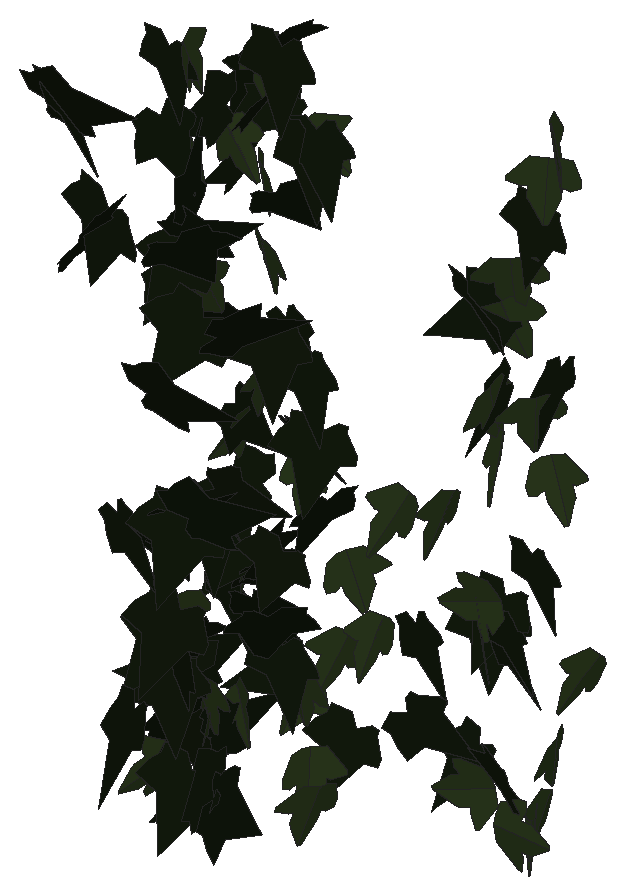
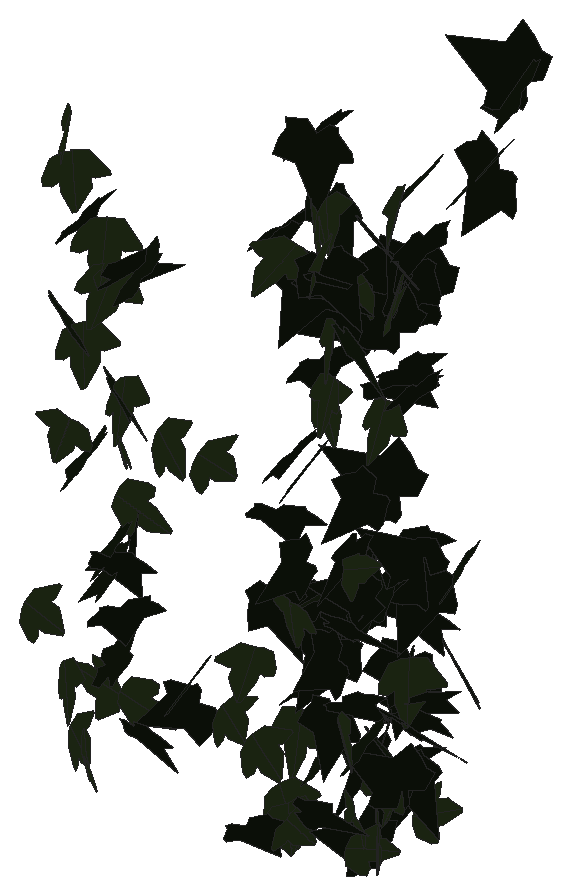
# SketchUp Ruby script. Lengths in inches.
U = 1.inch
M = Sketchup.active_model
def pt(a) = Geom::Point3d.new(a.map { |v| v * U })
def face(e, loops, mat)
  f = e.add_face(loops[0].map { |a| pt(a) })
  loops[1..].each { |l| e.add_face(l.map { |a| pt(a) }).erase! }
  f.material = f.back_material = mat if mat
  f
end
# faces: each face lists its corners as indices into pts; further lists are holes
def faces(e, pts, list, mat = nil) = list.each { |f| face(e, (f[0].is_a?(Array) ? f : [f]).map { |l| l.map { |i| pts[i] } }, mat) }
# xy, xz, yz: faces in a plane at the given z, y or x. An outline is a flat list of corners, or four numbers for a rectangle; further outlines are holes
def ring(l) = l.size == 4 ? [[l[0], l[1]], [l[2], l[1]], [l[2], l[3]], [l[0], l[3]]] : l.each_slice(2).to_a
def flat(e, list, mat, &to3) = list.each { |f| face(e, (f[0].is_a?(Array) ? f : [f]).map { |l| ring(l).map { |u, v| to3.(u, v) } }, mat) }
def xy(e, z, list, mat = nil) = flat(e, list, mat) { |x, y| [x, y, z] }
def xz(e, y, list, mat = nil) = flat(e, list, mat) { |x, z| [x, y, z] }
def yz(e, x, list, mat = nil) = flat(e, list, mat) { |y, z| [x, y, z] }
def lines(e, pts, list) = list.each { |a, b| e.add_line(pt(pts[a]), pt(pts[b])) }
# prism: a flat outline (further loops are holes) pulled along v
def prism(e, loops, v, mat = nil)
  f = face(e, loops, mat); d = Geom::Vector3d.new(v.map { |x| x * U })
  f.pushpull(f.normal.samedirection?(d) ? d.length : -d.length)
end
def box(e, o, s, mat = nil) = prism(e, [[o, [o[0] + s[0], o[1], o[2]], [o[0] + s[0], o[1] + s[1], o[2]], [o[0], o[1] + s[1], o[2]]]], [0, 0, s[2]], mat)
def at(x, y, z, deg = 0) = Geom::Transformation.translation(pt([x, y, z])) * Geom::Transformation.rotation(ORIGIN, Z_AXIS, deg.degrees)
def axes(o, x, y, z) = Geom::Transformation.new([*x, 0, *y, 0, *z, 0, *pt(o).to_a, 1])
def part(name) = M.definitions.add(name)
# library, detail: a bought-in or finely detailed component or shape, given as its bounding box
def library(name, o, s) = part(name).tap { |d| box(d.entities, o, s) }
def detail(e, o, s) = box(e.add_group.entities, o, s)
def put(e, d, t, mat = nil) = e.add_instance(d, t).tap { |i| i.material = mat if mat }
def group(e, t, mat = nil) = e.add_group.tap { |g| g.transformation = t; g.material = mat if mat }.entities
root = M.entities
M.materials.add("efeu1").color = [18, 25, 13]
M.materials.add("efeu2").color = [43, 57, 29]
c1 = part("ivyleaf_9")
p = [[1.54,2.16,1.25],[1.36,2.04,1.19],[-0.21,0.99,0.68],[-0.71,1.11,0.82],[-0.85,0.86,0.67],[-0.8,0.17,0.21],
  [-0.9,-0.01,0.1],[-0.67,-0.16,-0.02],[-0.08,-0.08,-0.05],[-0.03,-0.6,-0.4],[0.65,-0.88,-0.66],[0.83,-0.6,-0.49],
  [1.29,-0.42,-0.43],[1.8125,-0.07,-0.26],[1.21,0.44,0.15]]
faces(c1.entities,p,[[0,1,2,3,4,5,6,7,8,9,10,11,12,13,14]],"efeu1")
c2 = part("ivyleaf_10")
p = [[0,0.5,-0.03],[-0.0625,2.02,-0.43],[-0.19,2.01,-0.46],[-0.54,1.05,-0.29],[-0.52,0.625,-0.18],[-0.83,0.76,-0.28],
  [-1.16,0.64,-0.33],[-1.15,0.33,-0.24],[-0.77,-0.39,0.02],[-0.3,-0.51,0.16],[0.04,-0.48,0.23],[-0.02,2.01,-0.4375],
  [-0.06,2.01,-0.43],[0.04,-0.49,0.23],[0.67,-0.49,0.14],[1.38,0.36,-0.2],[1.375,0.51,-0.24],[0.81,0.65,-0.19],
  [0.62,0.59,-0.15],[0.6,1.09,-0.28],[0.5,1.23,-0.31]]
faces(c2.entities,p,[[0,1,2,3,4,5,6,7,8,9,10],[11,12,0,13,14,15,16,17,18,19,20]],"efeu2")
put(root,c1,axes([505.17,116.25,275.17],[0.52093,-0.38038,1.18336],[1.14923,-0.43079,-0.6189],[0.59847,1.15835,0.15843]))
put(root,c1,axes([506.65,117.58,270.4],[-0.10855,-1.09886,0.74671],[0.12021,-0.72463,-1.13718],[1.41254,-0.02278,0.15416]))
put(root,c1,axes([504.65,117.03,275.1],[0.77226,-0.95206,0.32614],[0.18154,-0.26586,-1.23805],[1.06724,0.73414,-0.0254]))
put(root,c1,axes([506.9375,115.67,270.03],[0.23492,1.04021,0.76758],[0.17346,0.72041,-1.10519],[-1.36652,0.27027,-0.00833]))
put(root,c1,axes([509.34,116.88,263.82],[0.67363,-0.32063,1.11659],[1.08327,-0.38796,-0.72651],[0.53942,1.17952,0.06457]))
put(root,c1,axes([506.99,118.65,248.56],[-1.05734,0.11517,-0.80677],[0.81643,-0.19168,-1.0218],[-0.22544,-1.23431,0.0834]))
put(root,c1,axes([508.26,120.65,256.49],[0.3412,-0.2438,1.2276],[1.23845,-0.31503,-0.38686],[0.40092,1.18062,0.15027]))
put(root,c1,axes([507.13,121.23,251.75],[-1.09872,-0.50946,-0.32223],[0.33647,0.06829,-1.18065],[0.54908,-1.06127,0.07871]))
put(root,c1,axes([507.28,121.79,244.67],[-0.50911,-1.02221,0.18292],[-0.05197,-0.17144,-1.17034],[1.119,-0.47303,0.02887]))
put(root,c1,axes([508.73,121.21,244.91],[-1.0834,0.6632,0.14675],[-0.1257,0.07982,-1.25066],[-0.72142,-1.00988,-0.00247]))
put(root,c1,axes([504.18,121.41,254.75],[0.73239,-0.84204,-0.25402],[-0.16045,0.19396,-1.12438],[0.93319,0.6942,0.00603]))
put(root,c1,axes([506.95,122.05,255.43],[-0.77344,-0.96925,-0.12279],[0.08584,0.08807,-1.25327],[1.05102,-0.72046,0.01199]))
put(root,c1,axes([509.58,120.73,264.65],[0.76725,0.40794,0.97112],[0.74256,0.64824,-0.83854],[-0.81224,0.97797,0.15074]))
put(root,c1,axes([507.34,121.01,267.73],[0.76991,1.02592,-0.02188],[-0.01175,-0.01805,-1.29926],[-1.10817,0.71296,-0.00142]))
put(root,c1,axes([509.17,120.96,244.51],[0.34449,-0.2086,-1.23135],[-0.81236,0.92096,-0.37949],[1.01288,0.80958,0.11443]))
put(root,c1,axes([505.78,122.6875,248.05],[-0.62327,-0.66376,-0.64536],[0.74275,0.16138,-0.8447],[0.64137,-0.83191,0.35107]))
put(root,c1,axes([506.74,123.05,263.35],[-0.90501,-0.82243,0.19368],[-0.0826,-0.18733,-1.21832],[0.90696,-0.83773,0.0823]))
put(root,c1,axes([506.62,121.84,249.64],[0.67569,-0.2485,-0.99126],[-0.8866,0.49246,-0.69393],[0.58789,1.02829,0.09278]))
put(root,c2,axes([504.74,123.16,243.67],[0.00953,-0.18123,1.04984],[0.07515,-1.00707,-0.18866],[1.1051,0.07005,0.00378]))
put(root,c1,axes([505.47,122.07,254.36],[0.56594,0.96324,-0.36059],[0.19221,0.29785,1.14033],[1.08881,-0.55326,-0.01388]))
put(root,c1,axes([505.34,122.18,254.23],[0.98085,0.6315,-0.27896],[-0.24823,-0.13925,-1.15029],[-0.69818,0.93668,0.01707]))
put(root,c1,axes([506.26,122.25,250.05],[0.42626,1.02562,-0.08071],[-0.0406,-0.06868,-1.14285],[-1.1101,0.39634,0.01081]))
put(root,c1,axes([504.98,123.66,249.13],[-0.76058,-0.74998,0.309],[-0.07526,-0.33638,-1.05482],[0.86797,-0.68635,0.17931]))
put(root,c1,axes([509.875,123.59,263.51],[-0.24528,-1.0606,-0.23525],[0.02896,0.2347,-1.08833],[1.08599,-0.24581,-0.02411]))
put(root,c1,axes([510.18,122.85,251.9],[0.43372,0.99156,-0.47764],[-0.27815,-0.38963,-1.10907],[-1.14693,0.46946,0.08835]))
put(root,c1,axes([504.54,123.9375,273.81],[0.22493,-0.99652,0.29595],[0.12298,-0.2665,-1.05724],[1.11249,0.23095,0.05704]))
put(root,c1,axes([506.13,123.44,247.83],[-0.92518,0.55615,0.58432],[-0.68246,0.0161,-1.01859],[-0.51304,-1.02433,0.30124]))
put(root,c1,axes([504.61,123.42,271.05],[0.25445,-0.88004,-0.63505],[-0.20014,0.60303,-0.91586],[1.06663,0.32309,-0.02036]))
put(root,c1,axes([505.1,124.3,265.1],[-0.55751,-0.91872,0.25014],[-0.12878,-0.21444,-1.07465],[0.94342,-0.57219,0.00112]))
put(root,c2,axes([509.52,123.77,262.03],[0.06793,-1.10361,0.0718],[0.00363,-0.07171,-1.1057],[1.10594,0.06802,-0.00078]))
put(root,c1,axes([505.9375,123.54,266.375],[0.21379,-0.32792,1.04485],[1.12351,-0.11963,-0.25378],[0.2011,1.01697,0.30706]))
put(root,c2,axes([505.22,123.6,250.46],[-0.70418,-0.88175,-0.08616],[0.0531,0.06668,-1.14051],[0.95501,-0.65387,-0.00012]))
put(root,c1,axes([505.07,123.68,246.02],[-0.25122,0.87354,-0.57099],[0.18593,-0.52206,-0.9397],[-1.09867,-0.28809,-0.02847]))
put(root,c1,axes([506.03,123.23,267.9],[-0.00768,-0.53438,1.00552],[0.38152,0.915,0.52865],[-1.13043,0.31245,0.17159]))
put(root,c1,axes([504.68,123.79,264.14],[0.3087,-0.86791,-0.47347],[-0.10042,0.44808,-0.94909],[1.0537,0.29697,0.04827]))
put(root,c2,axes([514.93,124.75,257.57],[-0.27825,-0.66374,0.83603],[0.13021,-0.87862,-0.65421],[1.0595,-0.06633,0.29997]))
put(root,c1,axes([506.04,124.69,253.84],[0.08578,-1.05034,0.19122],[0.04549,-0.18807,-1.05342],[1.06664,0.09249,0.02955]))
put(root,c1,axes([509.22,124.78,275.02],[-0.01952,-1.14955,0.07851],[0.00832,-0.07562,-1.19565],[1.24416,-0.01753,0.00923]))
put(root,c1,axes([504.9375,125.18,244.17],[-0.1907,-0.51831,0.88788],[-0.31551,-0.80225,-0.56937],[1.03148,-0.34122,-0.01001]))
put(root,c1,axes([508.94,125.18,253.21],[-0.38726,-0.9227,0.38725],[0.2551,-0.49255,-0.91849],[0.96761,-0.23943,0.39714]))
put(root,c1,axes([509.17,124.97,249.28],[0.04492,-1.10672,0.07115],[0.15309,-0.06259,-1.14269],[1.18771,0.04993,0.1446]))
put(root,c2,axes([516.73,125.23,258.07],[0.07718,-1.00594,0.46449],[0.10532,-0.45685,-1.00689],[1.10299,0.11401,0.06364]))
put(root,c1,axes([518.17,125.4,253.47],[0.235,-0.1964,-1.08534],[1.05881,-0.27069,0.27824],[-0.30897,-1.07699,0.12798]))
put(root,c2,axes([519.74,125.15,245.26],[0.03123,-0.01072,-1.17609],[1.07123,-0.48546,0.03287],[-0.48557,-1.07168,-0.00312]))
put(root,c1,axes([505.64,125.48,253.74],[0.91062,-0.42674,-0.39031],[0.37269,-0.14905,0.98256],[-0.48765,-0.9108,0.02208]))
put(root,c2,axes([510.55,125.14,243.39],[-0.33129,-1.02458,0.20946],[-0.09685,-0.18329,-1.11178],[1.12356,-0.31791,-0.03407]))
put(root,c1,axes([506.35,124.94,271.55],[-0.99273,0.49857,0.18309],[-0.16548,0.08676,-1.08752],[-0.54653,-0.93187,-0.00329]))
put(root,c1,axes([508.1875,124.53,251.23],[1.08341,0.46682,-0.15161],[-0.13946,-0.06801,-1.15069],[-0.50943,1.01141,-0.0074]))
put(root,c2,axes([504.86,124.73,273.42],[-0.36927,0.89214,0.47136],[-0.28914,0.37995,-0.98784],[-1.04133,-0.42186,0.10713]))
put(root,c2,axes([505.01,125.03,267.94],[-0.4526,0.92073,-0.14454],[-0.0838,0.11735,1.05183],[1.00215,0.42564,0.02267]))
put(root,c2,axes([518.66,125.22,254.54],[0.398,0.04113,-1.06387],[-1.04396,0.23796,-0.38136],[0.20893,1.11067,0.1211]))
put(root,c1,axes([519.09,125.89,246.6],[0.70387,-0.90274,0.01591],[-0.00607,0.01544,1.1447],[-0.90286,-0.70388,0.0047]))
put(root,c1,axes([509.73,125.82,270.9375],[0.11078,-1.0783,-0.01621],[-0.02104,0.0138,-1.12634],[1.1645,0.10283,-0.01881]))
put(root,c1,axes([508.18,125.01,272.47],[-0.34799,1.09799,-0.06976],[0.01748,-0.06515,-1.19006],[-1.18791,-0.3226,0.00293]))
put(root,c2,axes([504.89,125.47,246.07],[-1.07916,0.32487,-0.02481],[0.02883,0.00496,-1.09265],[-0.35062,-0.99949,-0.01348]))
put(root,c2,axes([505.17,125.3,263.43],[-0.21232,-0.86767,-0.56761],[0.15656,0.52661,-0.92498],[1.09592,-0.24333,0.02218]))
put(root,c1,axes([505.68,125.46,254.66],[0.47856,0.07305,-0.93544],[0.7345,0.6316,0.40179],[0.64061,-0.77875,0.23812]))
put(root,c1,axes([508.85,125.14,268.59],[0.81362,0.83167,0.02557],[0.01574,0.01997,-1.16703],[-0.89846,0.75349,0.00271]))
put(root,c1,axes([520.09,126.23,256.46],[0.43561,-0.99043,0.25411],[0.13106,-0.21985,-1.08156],[1.01407,0.45387,0.03063]))
put(root,c1,axes([508.73,125.28,275.21],[0.2458,1.09335,-0.13051],[-0.21198,-0.08577,-1.14735],[-1.16952,0.24534,0.18053]))
put(root,c1,axes([509.79,126.21,271.01],[0.06052,-1.10092,-0.11858],[0.12126,0.11923,-1.1399],[1.18918,0.04387,0.12227]))
put(root,c1,axes([503.79,125.62,246.4],[0.01727,-0.04178,1.08389],[1.11902,0.12043,-0.01151],[-0.12947,1.03535,0.04507]))
put(root,c2,axes([505.75,126.24,269.7],[-0.76922,-0.00916,-0.76445],[0.70434,-0.48014,-0.65098],[-0.36634,-0.9039,0.35354]))
put(root,c2,axes([517.79,125.98,245.9],[0.38776,-0.04236,-1.05479],[-1.03653,0.19758,-0.38898],[0.19996,1.1063,0.02908]))
put(root,c2,axes([509.2,125.94,247.72],[-1.13908,0.27295,0.15557],[-0.16415,0.00954,-1.13264],[-0.29335,-1.06522,0.02972]))
put(root,c1,axes([509.01,126.55,260.75],[0.21736,-1.05641,0.00052],[-0.00044,-0.00059,-1.11843],[1.14092,0.20126,-0.00053]))
put(root,c1,axes([517.98,127.06,266.07],[-0.6048,-0.46642,0.84272],[-0.60178,-0.59398,-0.76063],[0.75205,-0.85038,0.06907]))
put(root,c1,axes([509.62,126.69,257.89],[-0.76739,-0.74213,-0.34057],[0.34534,0.14384,-1.06056],[0.80512,-0.76904,0.13029]))
put(root,c1,axes([518.37,126.55,252.99],[0.568,-0.87512,0.10404],[0.06403,-0.08247,-1.04326],[0.87895,0.57153,0.00876]))
put(root,c1,axes([516.75,126.86,266.4375],[0.42626,-0.89452,0.54801],[0.38465,-0.41705,-0.97995],[0.97597,0.55505,0.14687]))
put(root,c2,axes([505.61,127,256.74],[-0.20781,0.35606,-0.91198],[-0.28127,-0.88022,-0.31227],[-0.98269,0.17664,0.28224]))
put(root,c2,axes([505.08,127.12,243.7],[-0.23128,-0.1376,0.94144],[-0.22195,-0.89871,-0.19263],[0.96365,-0.24002,0.18158]))
put(root,c2,axes([504.71,126.21,244.69],[0.44301,-0.76352,-0.53721],[-0.12313,0.54164,-0.87136],[0.92542,0.43757,0.14123]))
put(root,c2,axes([509.23,126.5,243.77],[0.43687,0.99145,-0.119],[-0.14938,-0.06658,-1.10852],[-1.06747,0.41507,0.10642]))
put(root,c1,axes([518.2,126.7,252.21],[0.73191,-0.74383,-0.06179],[-0.0401,0.04722,-1.04353],[0.74532,0.73299,0.00453]))
put(root,c2,axes([505.31,127.01,245],[0.60794,-0.27108,0.72641],[0.71967,-0.21824,-0.6466],[0.36991,0.87011,0.06413]))
put(root,c2,axes([519.8,126.79,262.6],[-0.62345,-0.89179,-0.00734],[0.00421,0.00601,-1.08811],[0.89181,-0.62347,0.00001]))
put(root,c2,axes([506.66,127.11,273.23],[0.00982,-1.01358,0.20743],[0.34003,-0.18725,-1.00457],[1.06258,0.06928,0.31955]))
put(root,c1,axes([504.88,126.24,243.56],[0.11095,0.11,1.08915],[0.94265,0.57974,-0.15237],[-0.63621,0.87818,-0.03583]))
put(root,c2,axes([518.54,126.95,268.01],[-0.91203,-0.69038,-0.05057],[0.04556,0.0236,-1.14383],[0.69073,-0.91312,0.00867]))
put(root,c1,axes([513.83,126.76,247.33],[0.10243,-0.10547,-1.05394],[0.63557,0.85316,-0.02361],[0.84732,-0.62721,0.14512]))
put(root,c1,axes([520.17,127.7,263.82],[-0.65571,-0.2797,-0.82476],[0.8691,-0.27643,-0.59722],[-0.05591,-1.01675,0.38925]))
put(root,c1,axes([505.59,126.69,257.6875],[0.34857,-0.41462,-0.85743],[-0.44206,0.71849,-0.54243],[0.89327,0.51736,0.06615]))
put(root,c2,axes([506.77,126.95,264.74],[-0.92365,0.50957,0.1431],[-0.12747,0.07073,-1.03535],[-0.55561,-0.86334,-0.00036]))
put(root,c1,axes([517.56,127.63,253.24],[-0.85302,-0.5552,-0.24044],[0.21091,0.11667,-1.01765],[0.56708,-0.87855,0.01681]))
put(root,c2,axes([518.16,127.05,265.99],[-0.79793,-0.71473,-0.37085],[0.33494,0.18018,-1.0679],[0.73225,-0.86125,0.08435]))
put(root,c1,axes([506.83,126.39,251.69],[0.20947,0.55778,0.85239],[0.35278,0.75256,-0.61303],[-1.01093,0.37819,-0.0373]))
put(root,c1,axes([506,127.49,254.15],[-0.85067,0.24391,0.50482],[-0.55364,-0.05079,-0.83857],[-0.19416,-0.92382,0.17939]))
put(root,c1,axes([504.11,127.82,249.24],[0.43441,-0.92401,0.26752],[0.14601,-0.22153,-1.04746],[1.02554,0.42294,0.03582]))
put(root,c1,axes([509.29,127.42,254.49],[-0.19019,0.86362,-0.60756],[0.12678,-0.57227,-0.91665],[-1.1189,-0.21164,-0.00059]))
put(root,c2,axes([507.16,127.36,272.9],[0.7544,-0.73432,-0.19341],[-0.00244,0.25096,-1.03935],[0.8181,0.67789,0.17526]))
put(root,c2,axes([508.97,126.89,270.33],[0.44793,0.69658,0.74775],[0.24752,0.69151,-0.83425],[-1.05245,0.4591,0.12204]))
put(root,c1,axes([504.99,128.0625,251.07],[-0.74694,-0.58549,0.18683],[-0.11819,-0.14847,-0.9414],[0.65078,-0.69897,0.04346]))
put(root,c2,axes([517.03,127.92,259.47],[0.77224,-0.65183,0.47638],[0.37031,-0.29981,-1.01052],[0.71742,0.85639,0.00882]))
put(root,c1,axes([506.15,128.08,247.79],[0.14941,-0.84372,0.39731],[0.1774,-0.35779,-0.88366],[0.98441,0.19253,0.09894]))
put(root,c2,axes([506.31,127.37,267.71],[-0.74947,0.69639,0.24192],[-0.24906,0.09714,-1.01794],[-0.75282,-0.72542,0.09593]))
put(root,c1,axes([505.37,127.48,267.9],[-0.74659,0.69844,0.0884],[-0.08282,0.04365,-1.02171],[-0.75536,-0.69512,0.02466]))
put(root,c1,axes([507.16,127.74,261.41],[0.52052,-0.83263,-0.22984],[-0.11066,0.19604,-1.00049],[0.92377,0.49264,0.00966]))
put(root,c2,axes([519,128.23,244.71],[0.2766,-0.87809,0.5509],[0.3077,-0.47492,-0.91148],[0.98987,0.39299,0.1294]))
put(root,c1,axes([515.87,128.13,246.05],[-0.98834,-0.15828,-0.18142],[0.18423,-0.00368,-1.00042],[0.15501,-1.00485,0.03224]))
put(root,c1,axes([504.2,127.39,260.86],[1.00952,0.22113,0.03484],[0.0367,0.00189,-0.99895],[-0.23874,0.93534,-0.00622]))
put(root,c2,axes([518.42,128.31,243.875],[0.63598,-0.53135,0.67206],[0.54256,-0.39797,-0.82808],[0.66305,0.83531,0.03298]))
put(root,c2,axes([516.78,127.82,261.5],[-0.03914,-1.06551,-0.32741],[0.17807,0.31742,-1.05431],[1.10036,-0.08927,0.15898]))
put(root,c1,axes([517.1,128.21,261.85],[-0.91163,0.32366,-0.47038],[0.44119,-0.16321,-0.96736],[-0.36244,-1.01276,0.00557]))
put(root,c1,axes([506.4375,128.45,270.48],[-1.03306,-0.25869,0.26078],[-0.24713,-0.11324,-1.02933],[0.30053,-0.98236,0.04999]))
put(root,c1,axes([518.4375,128.72,269.44],[-0.08498,-1.04011,0.36056],[0.00135,-0.36173,-1.04317],[1.10083,-0.07985,0.02911]))
put(root,c1,axes([507.25,127.96,256.8125],[1.01326,-0.212,-0.01092],[-0.01054,0.00444,-1.00033],[0.229,0.93825,0.00226]))
put(root,c2,axes([509.09,128.63,247.89],[-0.35211,-0.81136,0.5472],[0.00663,-0.55697,-0.88929],[1.04436,-0.27002,0.19013]))
put(root,c1,axes([505.8,128.22,271.57],[0.34107,0.48797,-0.88868],[-0.53352,-0.69752,-0.60414],[-0.91911,0.58597,0.02091]))
put(root,c2,axes([519.55,128.16,247.36],[0.2386,-0.97163,-0.25209],[-0.00171,0.25872,-0.9988],[1.0038,0.2314,0.05822]))
put(root,c2,axes([519.43,128.23,259.12],[0.9573,0.21211,0.42187],[0.39595,0.15903,-0.97843],[-0.25728,1.03398,0.06394]))
put(root,c2,axes([519.04,128.47,271.7],[-0.84362,-0.71578,0.12035],[0.08262,-0.27804,-1.07442],[0.72111,-0.80553,0.26391]))
put(root,c1,axes([516.25,128.72,251.8125],[-0.39375,-0.97676,-0.27931],[0.12227,0.25182,-1.05297],[1.00853,-0.41187,0.01861]))
put(root,c2,axes([510.53,128.86,248.93],[-0.25177,-0.79469,0.57239],[0.22039,-0.59385,-0.80187],[1.02047,-0.06781,0.3144]))
put(root,c2,axes([507.39,128.49,254.82],[0.99712,-0.18449,0.15846],[0.16377,-0.01865,-0.97911],[0.1999,0.93557,0.01173]))
put(root,c1,axes([509.375,128.93,244.1],[-0.72125,-0.73818,-0.00781],[0.00313,0.0075,-1.03525],[0.79727,-0.66783,-0.003]))
put(root,c2,axes([519.4375,128.33,273.42],[-0.62881,0.92464,-0.04747],[-0.07316,-0.10683,-1.11169],[-0.92296,-0.62149,0.12046]))
put(root,c2,axes([505.99,128.16,272.15],[-0.42205,0.93785,0.20343],[-0.05848,0.1893,-1.05639],[-1.03302,-0.39388,-0.02331]))
put(root,c2,axes([504.7,128.6,250.1875],[0.48008,-0.80102,-0.02036],[-0.00668,0.01896,-0.95273],[0.86534,0.44455,0.00394]))
put(root,c1,axes([506.48,128.88,245.76],[-0.83136,-0.08084,0.50861],[-0.52305,-0.06979,-0.8048],[0.11406,-0.90932,0.01655]))
put(root,c1,axes([505.58,128.04,250.27],[0.22626,0.91299,0.04653],[0.01425,0.04287,-0.97418],[-0.98711,0.20989,-0.00339]))
put(root,c2,axes([509.71,128.27,251.67],[0.66274,0.73935,0.32165],[0.05029,0.35598,-0.98111],[-0.86408,0.58779,0.1896]))
put(root,c1,axes([512.51,128.78,249.74],[0.53731,-0.91059,-0.11841],[-0.06872,0.09693,-1.05725],[0.91568,0.5416,-0.00987]))
put(root,c2,axes([520.375,129.27,250.625],[-0.04715,-0.74746,0.72575],[0.01295,-0.72686,-0.74776],[1.04175,-0.0248,0.04214]))
put(root,c2,axes([507.07,129.01,245.08],[0.3283,0.64745,-0.603],[-0.29179,-0.51343,-0.74356],[-0.89214,0.40617,0.02129]))
